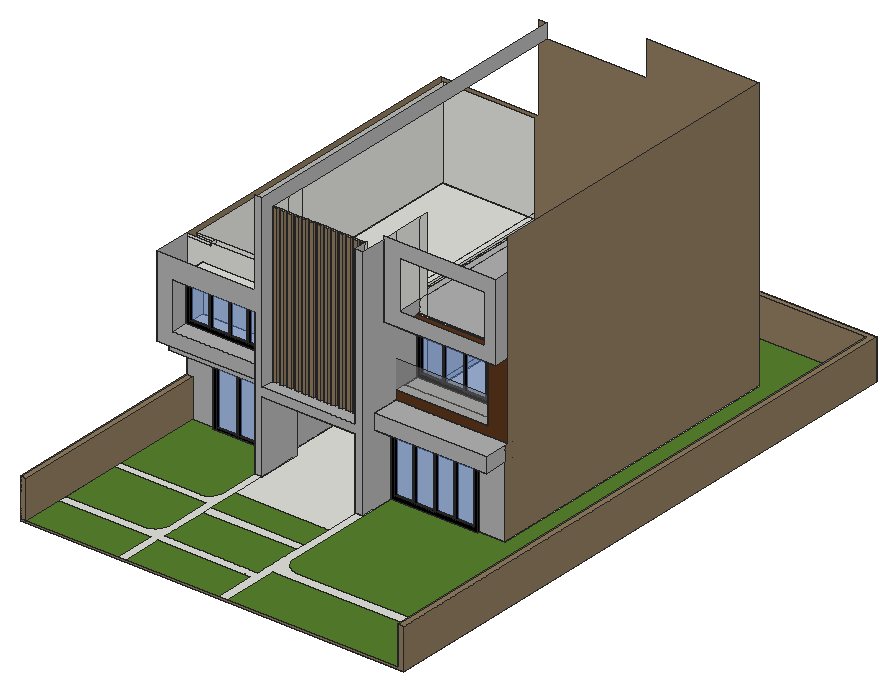
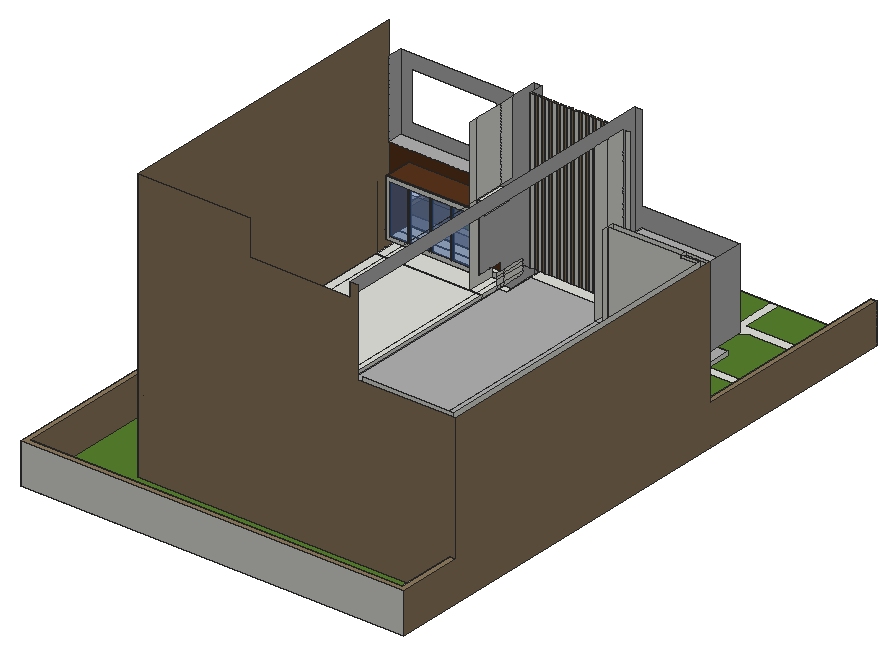
# SketchUp Ruby script. Lengths in inches.
U = 1.inch
M = Sketchup.active_model
def pt(a) = Geom::Point3d.new(a.map { |v| v * U })
def face(e, loops, mat)
  f = e.add_face(loops[0].map { |a| pt(a) })
  loops[1..].each { |l| e.add_face(l.map { |a| pt(a) }).erase! }
  f.material = f.back_material = mat if mat
  f
end
# faces: each face lists its corners as indices into pts; further lists are holes
def faces(e, pts, list, mat = nil) = list.each { |f| face(e, (f[0].is_a?(Array) ? f : [f]).map { |l| l.map { |i| pts[i] } }, mat) }
# xy, xz, yz: faces in a plane at the given z, y or x. An outline is a flat list of corners, or four numbers for a rectangle; further outlines are holes
def ring(l) = l.size == 4 ? [[l[0], l[1]], [l[2], l[1]], [l[2], l[3]], [l[0], l[3]]] : l.each_slice(2).to_a
def flat(e, list, mat, &to3) = list.each { |f| face(e, (f[0].is_a?(Array) ? f : [f]).map { |l| ring(l).map { |u, v| to3.(u, v) } }, mat) }
def xy(e, z, list, mat = nil) = flat(e, list, mat) { |x, y| [x, y, z] }
def xz(e, y, list, mat = nil) = flat(e, list, mat) { |x, z| [x, y, z] }
def yz(e, x, list, mat = nil) = flat(e, list, mat) { |y, z| [x, y, z] }
def lines(e, pts, list) = list.each { |a, b| e.add_line(pt(pts[a]), pt(pts[b])) }
# prism: a flat outline (further loops are holes) pulled along v
def prism(e, loops, v, mat = nil)
  f = face(e, loops, mat); d = Geom::Vector3d.new(v.map { |x| x * U })
  f.pushpull(f.normal.samedirection?(d) ? d.length : -d.length)
end
def box(e, o, s, mat = nil) = prism(e, [[o, [o[0] + s[0], o[1], o[2]], [o[0] + s[0], o[1] + s[1], o[2]], [o[0], o[1] + s[1], o[2]]]], [0, 0, s[2]], mat)
def at(x, y, z, deg = 0) = Geom::Transformation.translation(pt([x, y, z])) * Geom::Transformation.rotation(ORIGIN, Z_AXIS, deg.degrees)
def axes(o, x, y, z) = Geom::Transformation.new([*x, 0, *y, 0, *z, 0, *pt(o).to_a, 1])
def part(name) = M.definitions.add(name)
# library, detail: a bought-in or finely detailed component or shape, given as its bounding box
def library(name, o, s) = part(name).tap { |d| box(d.entities, o, s) }
def detail(e, o, s) = box(e.add_group.entities, o, s)
def put(e, d, t, mat = nil) = e.add_instance(d, t).tap { |i| i.material = mat if mat }
def group(e, t, mat = nil) = e.add_group.tap { |g| g.transformation = t; g.material = mat if mat }.entities
root = M.entities
M.materials.add("Niraj_Hair_Gray").color = [178, 178, 178]
M.materials.add("[0035_Tan]").color = [142, 122, 95]
M.materials.add("[0137_Black]").color = [0, 0, 0]
M.materials.add("[Grass Dark Green]").color = [87, 130, 45]
M.materials.add("[Translucent Glass Blue]").color = [100, 149, 237]
M.materials["[Translucent Glass Blue]"].alpha = 0.5
M.materials.add("[Translucent Glass Gray]").color = [128, 128, 128]
M.materials["[Translucent Glass Gray]"].alpha = 0.5
M.materials.add("[Wood Veneer 01]").color = [89, 52, 27]
xy(root,0,[[0,0,0,325.73,43.58,325.73,43.58,322.73,152.61,322.73,152.61,267.73,164.61,267.73,164.61,334.73,152.61,334.73,152.61,814.73,322.3125,814.73,322.3125,334.73,310.3125,334.73,310.3125,267.73,322.3125,267.73,322.3125,325.73,498,325.73,498,823.73,0,823.73,0,925.52,599.79,925.52,599.79,0],[152.61,267.73,164.61,289.73],[310.3125,267.73,322.3125,289.73],[152.61,289.73,164.61,325.73],[310.3125,289.73,322.3125,325.73],
  [43.58,322.73,152.61,325.73],[0,325.73,0,823.73,498,823.73,498,325.73,322.3125,325.73,322.3125,334.73,489,334.73,489,814.73,9,814.73,9,334.73,152.61,334.73,152.61,325.73],[152.61,325.73,164.61,334.73],[310.3125,325.73,322.3125,334.73],[9,334.73,152.61,814.73],
  [322.3125,334.73,489,814.73]])
xy(root,3,[[152.61,0,164.5625,0,164.5625,63.91,310.3125,63.91,310.3125,0,322.96,0,322.96,90.65,590.79,90.65,590.79,105.17,349.55,105.17,346.08,105.39,342.67,106.07,339.38,107.19,336.26,108.73,333.37,110.66,330.75,112.96,328.46,115.57,326.52,118.46,324.99,121.58,323.87,124.88,323.1875,128.29,322.96,131.76,322.96,267.73,310.3125,267.73,310.3125,76.4,164.5625,76.4,164.5625,267.73,152.61,267.73,152.61,206.62,152.43,203.89,151.9,201.2,151.02,198.61,149.8125,196.16,148.29,193.89,146.49,191.83,144.43,190.03,142.16,188.51,139.7,187.3,137.11,186.42,134.43,185.89,131.7,185.71,9,185.71,9,172.8,152.61,172.8,152.61,104.46,152.39,101.12,151.74,97.83,150.66,94.65,149.18,91.64,147.3125,88.85,145.1,86.33,142.58,84.11,139.79,82.25,136.78,80.77,133.6,79.6875,130.31,79.03,126.96,78.8125,9,78.8125,9,63.91,152.61,63.91],[306.22,63.75,310.3125,63.91,300.72,63.91,302.13,63.82],[164.5625,152.8,310.3125,166.42],[164.5625,215.1875,310.3125,215.1875,310.3125,334.73,322.3125,334.73,322.3125,814.73,152.61,814.73,152.61,334.73,164.61,334.73,164.61,267.73,164.5625,267.73],[322.3125,322.73,457.59,325.73]])
xy(root,3,[[9,0,152.61,63.91],[164.5625,0,310.3125,0,310.3125,63.91,306.22,63.75,302.13,63.82,300.72,63.91,164.5625,63.91],[322.96,0,590.79,90.65],[164.5625,76.4,310.3125,152.8],[9,78.8125,126.96,78.8125,130.31,79.03,133.6,79.6875,136.78,80.77,139.79,82.25,142.58,84.11,145.1,86.33,147.3125,88.85,149.18,91.64,150.66,94.65,151.74,97.83,152.39,101.12,152.61,104.46,152.61,172.8,9,172.8],
  [349.55,105.17,590.79,105.17,590.79,916.52,9,916.52,9,823.73,498,823.73,498,325.73,457.59,325.73,457.59,322.73,322.3125,322.73,322.3125,267.73,322.96,267.73,322.96,131.76,323.1875,128.29,323.87,124.88,324.99,121.58,326.52,118.46,328.46,115.57,330.75,112.96,333.37,110.66,336.26,108.73,339.38,107.19,342.67,106.07,346.08,105.39],[164.5625,166.42,310.3125,215.1875],[9,185.71,131.7,185.71,134.43,185.89,137.11,186.42,139.7,187.3,142.16,188.51,144.43,190.03,146.49,191.83,148.29,193.89,149.8125,196.16,151.02,198.61,151.9,201.2,152.43,203.89,152.61,206.62,152.61,322.73,43.58,322.73,43.58,325.73,9,325.73]],"[Grass Dark Green]")
xy(root,6,[[49.58,322.73,81.37,325.73],[84.37,322.73,116.66,325.73],[119.66,322.73,146.61,325.73]],"[0137_Black]")
xy(root,9,[[328.3125,322.73,356.625,325.73],[359.625,322.73,389.95,325.73],[392.95,322.73,421.03,325.73],[424.03,322.73,451.59,325.73]],"[0137_Black]")
xy(root,63,[[0,0,9,325.73],[590.79,0,599.79,0,599.79,925.52,0,925.52,0,823.73,9,823.73,9,916.52,590.79,916.52]],"[0035_Tan]")
xy(root,107.16,[[49.58,322.73,81.37,325.73],[84.37,322.73,116.66,325.73],[119.66,322.73,146.61,325.73]],"[0137_Black]")
xy(root,108.75,[[328.3125,322.73,356.625,325.73],[359.625,322.73,389.95,325.73],[392.95,322.73,421.03,325.73],[424.03,322.73,451.59,325.73]],"[0137_Black]")
xy(root,113.16,[[43.58,322.73,152.61,325.73]])
xy(root,113.16,[[0,289.73,0,325.73,43.58,325.73,43.58,322.73,152.61,322.73,152.61,289.73]],"Niraj_Hair_Gray")
xy(root,113.5,[[322.3125,334.73,489,369.1]])
xy(root,114.5625,[[164.61,267.73,310.3125,289.73],[152.61,325.73,164.61,334.73],[310.3125,325.73,322.3125,334.73]])
xy(root,114.5625,[[164.61,289.73,164.61,334.73,152.61,334.73,152.61,814.73,322.3125,814.73,322.3125,334.73,310.3125,334.73,310.3125,289.73]],"Niraj_Hair_Gray")
xy(root,114.75,[[322.3125,322.73,457.59,325.73]])
xy(root,114.75,[[322.3125,289.73,322.3125,322.73,457.59,322.73,457.59,325.73,498,325.73,498,289.73]],"Niraj_Hair_Gray")
xy(root,120,[[322.3125,325.73,489,369.1],[9,334.73,151.88,814.73],[322.3125,369.1,489,814.73]])
xy(root,120,[[0,289.73,152.61,325.73]],"Niraj_Hair_Gray")
xy(root,128.125,[[165.47,286.73,172.3125,289.73],[176.97,286.73,183.8125,289.73],[188.47,286.73,195.3125,289.73],[199.97,286.73,206.8125,289.73],[211.47,286.73,218.3125,289.73],
  [222.97,286.73,229.8125,289.73],[234.47,286.73,241.3125,289.73],[245.97,286.73,252.8125,289.73],[257.47,286.73,264.3125,289.73],[268.97,286.73,275.8125,289.73],
  [280.47,286.73,287.3125,289.73],[291.97,286.73,298.8125,289.73],[303.47,286.73,310.3125,289.73]])
xy(root,128.125,[[164.61,267.73,310.3125,267.73,310.3125,286.73,303.47,286.73,303.47,289.73,298.8125,289.73,298.8125,286.73,291.97,286.73,291.97,289.73,287.3125,289.73,287.3125,286.73,280.47,286.73,280.47,289.73,275.8125,289.73,275.8125,286.73,268.97,286.73,268.97,289.73,264.3125,289.73,264.3125,286.73,257.47,286.73,257.47,289.73,252.8125,289.73,252.8125,286.73,245.97,286.73,245.97,289.73,241.3125,289.73,241.3125,286.73,234.47,286.73,234.47,289.73,229.8125,289.73,229.8125,286.73,222.97,286.73,222.97,289.73,218.3125,289.73,218.3125,286.73,211.47,286.73,211.47,289.73,206.8125,289.73,206.8125,286.73,199.97,286.73,199.97,289.73,195.3125,289.73,195.3125,286.73,188.47,286.73,188.47,289.73,183.8125,289.73,183.8125,286.73,176.97,286.73,176.97,289.73,172.3125,289.73,172.3125,286.73,165.47,286.73,165.47,289.73,164.61,289.73]],"Niraj_Hair_Gray")
xy(root,135.375,[[0,267.73,152.61,325.73]],"Niraj_Hair_Gray")
xy(root,137.94,[[322.3125,332.48,466.55,339.92],[322.3125,349.98,466.55,392.92]])
xy(root,137.94,[[322.3125,289.73,498,332.48]],"Niraj_Hair_Gray")
xy(root,151.32,[[322.3125,332.48,466.55,349.98],[322.3125,349.98,466.55,373.98],[322.3125,373.98,466.55,376.98]])
xy(root,157.07,[[24.625,294.04,152.61,297.04],[24.625,297.04,152.61,325.73]])
xy(root,157.07,[[24.625,267.73,152.61,294.04]],"Niraj_Hair_Gray")
xy(root,157.32,[[328.3125,373.98,362.38,376.98],[365.38,373.98,394.43,376.98],[397.43,373.98,429.41,376.98],[432.41,373.98,460.55,376.98]],"[0137_Black]")
xy(root,163.07,[[30.625,294.04,60.5,297.04],[63.5,294.04,91.1875,297.04],[94.1875,294.04,119.75,297.04],[122.75,294.04,146.61,297.04]],"[0137_Black]")
xy(root,223.39,[[30.625,294.04,60.5,297.04],[63.5,294.04,91.1875,297.04],[94.1875,294.04,119.75,297.04],[122.75,294.04,146.61,297.04]],"[0137_Black]")
xy(root,229.39,[[24.625,294.04,152.61,297.04],[24.625,297.04,152.61,325.73]])
xy(root,229.39,[[24.625,267.73,152.61,294.04]],"Niraj_Hair_Gray")
xy(root,234,[[328.3125,373.98,362.38,376.98],[365.38,373.98,394.43,376.98],[397.43,373.98,429.41,376.98],[432.41,373.98,460.55,376.98]],"[0137_Black]")
xy(root,240,[[322.3125,373.98,466.55,376.98]])
xy(root,240,[[322.3125,332.48,466.55,373.98]],"[Wood Veneer 01]")
xy(root,240.1,[[309.68,332.48,322.3125,379.48]])
xy(root,257.94,[[309.68,332.48,322.3125,379.48]])
xy(root,257.94,[[322.3125,308.48,498,332.48]],"Niraj_Hair_Gray")
xz(root,0,[[0,0,599.79,0,599.79,63,590.79,63,590.79,3,0,3],[0,3,9,63]],"[0035_Tan]")
xz(root,267.73,[[152.61,0,164.61,3],[310.3125,0,322.3125,3]])
xz(root,267.73,[[152.61,3,164.61,3,164.61,114.5625,310.3125,114.5625,310.3125,3,322.3125,3,322.3125,372.875,310.3125,372.875,310.3125,128.125,164.61,128.125,164.61,394.4375,152.61,394.4375,152.61,261.125,0,261.125,0,135.375,152.61,135.375,152.61,157.07,24.625,157.07,24.625,229.39,152.61,229.39]],"Niraj_Hair_Gray")
xz(root,286.73,[[165.47,128.125,172.3125,372.875],[176.97,128.125,183.8125,372.875],[188.47,128.125,195.3125,372.875],[199.97,128.125,206.8125,372.875],[211.47,128.125,218.3125,372.875],
  [222.97,128.125,229.8125,372.875],[234.47,128.125,241.3125,372.875],[245.97,128.125,252.8125,372.875],[257.47,128.125,264.3125,372.875],[268.97,128.125,275.8125,372.875],
  [280.47,128.125,287.3125,372.875],[291.97,128.125,298.8125,372.875],[303.47,128.125,310.3125,372.875]],"[0035_Tan]")
xz(root,289.73,[[153.97,128.125,160.8125,372.875],[165.47,128.125,172.3125,372.875],[176.97,128.125,183.8125,372.875],[188.47,128.125,195.3125,372.875],[199.97,128.125,206.8125,372.875],
  [211.47,128.125,218.3125,372.875],[222.97,128.125,229.8125,372.875],[234.47,128.125,241.3125,372.875],[245.97,128.125,252.8125,372.875],[257.47,128.125,264.3125,372.875],
  [268.97,128.125,275.8125,372.875],[280.47,128.125,287.3125,372.875],[291.97,128.125,298.8125,372.875],[303.47,128.125,310.3125,372.875]])
xz(root,289.73,[[0,113.16,152.61,120],[322.3125,114.75,498,137.94]],"Niraj_Hair_Gray")
xz(root,289.73,[[164.61,128.125,165.47,372.875],[172.3125,128.125,176.97,372.875],[183.8125,128.125,188.47,372.875],[195.3125,128.125,199.97,372.875],[206.8125,128.125,211.47,372.875],
  [218.3125,128.125,222.97,372.875],[229.8125,128.125,234.47,372.875],[241.3125,128.125,245.97,372.875],[252.8125,128.125,257.47,372.875],[264.3125,128.125,268.97,372.875],
  [275.8125,128.125,280.47,372.875],[287.3125,128.125,291.97,372.875],[298.8125,128.125,303.47,372.875]],"[0035_Tan]")
xz(root,294.04,[[[24.625,157.07,152.61,229.39],[30.625,163.07,60.5,223.39],[63.5,163.07,91.1875,223.39],[94.1875,163.07,119.75,223.39],[122.75,163.07,146.61,223.39]]],"[0137_Black]")
xz(root,297.04,[[[24.625,157.07,152.61,229.39],[30.625,163.07,60.5,223.39],[63.5,163.07,91.1875,223.39],[94.1875,163.07,119.75,223.39],[122.75,163.07,146.61,223.39]]])
xz(root,297.04,[[30.625,163.07,60.5,223.39],[63.5,163.07,91.1875,223.39],[94.1875,163.07,119.75,223.39],[122.75,163.07,146.61,223.39]],"[Translucent Glass Blue]")
xz(root,308.48,[[[322.3125,257.94,498,377.94],[346.71,279.54,480.7,355.07]]],"Niraj_Hair_Gray")
xz(root,322.73,[[43.58,0,152.61,3]])
xz(root,322.73,[[[43.58,3,152.61,113.16],[84.37,6,116.66,107.16],[49.58,6,81.37,107.16],[119.66,6,146.61,107.16]],[[322.3125,3,457.59,114.75],[359.625,9,389.95,108.75],[328.3125,9,356.625,108.75],[392.95,9,421.03,108.75],[424.03,9,451.59,108.75]]],"[0137_Black]")
xz(root,325.73,[[[43.58,0,152.61,113.16],[84.37,6,116.66,107.16],[49.58,6,81.37,107.16],[119.66,6,146.61,107.16]],[322.3125,0,498,3],[[322.3125,3,457.59,114.75],[359.625,9,389.95,108.75],[328.3125,9,356.625,108.75],[392.95,9,421.03,108.75],[424.03,9,451.59,108.75]],[0,113.16,152.61,120],[322.3125,114.75,489,120],
  [489,114.75,498,120],[322.3125,120,498,132.82],[0,135.375,0,257.3125,38.3125,257.3125,38.3125,261.125,152.61,261.125,152.61,229.39,24.625,229.39,24.625,157.07,152.61,157.07,152.61,135.375],[0,257.3125,38.3125,261.125]])
xz(root,325.73,[[9,3,43.58,3,43.58,113.16,0,113.16,0,63,9,63],[457.59,3,498,114.75],[0,120,152.61,135.375]],"Niraj_Hair_Gray")
xz(root,325.73,[[49.58,6,81.37,107.16],[84.37,6,116.66,107.16],[119.66,6,146.61,107.16],[328.3125,9,356.625,108.75],[359.625,9,389.95,108.75],
  [392.95,9,421.03,108.75],[424.03,9,451.59,108.75]],"[Translucent Glass Blue]")
xz(root,332.48,[[322.3125,151.32,466.55,195.66]],"[Translucent Glass Gray]")
xz(root,332.48,[[322.3125,137.94,498,137.94,498,257.94,309.68,257.94,309.68,240.1,322.3125,240.1,322.3125,240,466.55,240,466.55,151.32,322.3125,151.32]],"[Wood Veneer 01]")
xz(root,334.73,[[9,0,9,120,151.88,120,151.88,261.125,152.61,261.125,152.61,0],[152.61,0,164.61,3],[310.3125,0,322.3125,3],[322.3125,0,489,113.5],[152.61,3,164.61,114.5625],
  [9,120,9,257.3125,38.3125,257.3125,38.3125,261.125,151.88,261.125,151.88,120],[9,257.3125,38.3125,261.125]])
xz(root,334.73,[[310.3125,3,322.3125,114.5625]],"Niraj_Hair_Gray")
xz(root,349.98,[[322.3125,137.94,466.55,151.32]])
xz(root,369.1,[[322.3125,113.5,489,120]])
xz(root,373.98,[[[322.3125,151.32,466.55,240],[328.3125,157.32,362.38,234],[397.43,157.32,429.41,234],[365.38,157.32,394.43,234],[432.41,157.32,460.55,234]]],"[0137_Black]")
xz(root,376.98,[[[322.3125,151.32,466.55,240],[328.3125,157.32,362.38,234],[397.43,157.32,429.41,234],[365.38,157.32,394.43,234],[432.41,157.32,460.55,234]]])
xz(root,376.98,[[328.3125,157.32,362.38,234],[365.38,157.32,394.43,234],[397.43,157.32,429.41,234],[432.41,157.32,460.55,234]],"[Translucent Glass Blue]")
xz(root,379.48,[[309.68,240.1,322.3125,257.94]])
xz(root,814.73,[[9,0,152.61,120],[152.61,0,322.3125,3],[322.3125,0,489,120],[152.61,114.5625,322.3125,120],[9,120,151.88,261.125]])
xz(root,814.73,[[152.61,3,322.3125,114.5625]],"Niraj_Hair_Gray")
xz(root,823.73,[[9,3,9,63,0,63,0,261.125,152.61,261.125,152.61,394.4375,164.61,394.4375,164.61,372.875,322.3125,372.875,322.3125,428.22,498,428.22,498,3]],"[0035_Tan]")
xz(root,916.52,[[9,3,590.79,63]],"[0035_Tan]")
xz(root,925.52,[[0,0,599.79,63]])
yz(root,0,[[289.73,113.16,325.73,120]])
yz(root,0,[[267.73,135.375,325.73,261.125]],"Niraj_Hair_Gray")
yz(root,0,[[0,0,0,63,325.73,63,325.73,261.125,823.73,261.125,823.73,63,925.52,63,925.52,0]],"[0035_Tan]")
yz(root,9,[[334.73,0,814.73,120],[823.73,3,916.52,63],[334.73,120,814.73,261.125]])
yz(root,9,[[0,3,325.73,63]],"[0035_Tan]")
yz(root,24.625,[[294.04,157.07,297.04,229.39],[297.04,157.07,325.73,229.39]])
yz(root,24.625,[[267.73,157.07,294.04,229.39]],"Niraj_Hair_Gray")
yz(root,30.625,[[294.04,163.07,297.04,223.39]],"[0137_Black]")
yz(root,38.3125,[[325.73,257.3125,334.73,261.125]])
yz(root,43.58,[[322.73,0,325.73,3]])
yz(root,43.58,[[322.73,3,325.73,113.16]],"[0137_Black]")
yz(root,49.58,[[322.73,6,325.73,107.16]],"[0137_Black]")
yz(root,60.5,[[294.04,163.07,297.04,223.39]],"[0137_Black]")
yz(root,63.5,[[294.04,163.07,297.04,223.39]],"[0137_Black]")
yz(root,81.37,[[322.73,6,325.73,107.16]],"[0137_Black]")
yz(root,84.37,[[322.73,6,325.73,107.16]],"[0137_Black]")
yz(root,91.1875,[[294.04,163.07,297.04,223.39]],"[0137_Black]")
yz(root,94.1875,[[294.04,163.07,297.04,223.39]],"[0137_Black]")
yz(root,116.66,[[322.73,6,325.73,107.16]],"[0137_Black]")
yz(root,119.66,[[322.73,6,325.73,107.16]],"[0137_Black]")
yz(root,119.75,[[294.04,163.07,297.04,223.39]],"[0137_Black]")
yz(root,122.75,[[294.04,163.07,297.04,223.39]],"[0137_Black]")
yz(root,146.61,[[322.73,6,325.73,107.16],[294.04,163.07,297.04,223.39]],"[0137_Black]")
yz(root,152.61,[[267.73,0,289.73,3],[289.73,0,322.73,3],[322.73,0,325.73,113.16],[325.73,0,334.73,114.5625],[334.73,0,814.73,3],
  [289.73,113.16,325.73,114.5625],[289.73,114.5625,325.73,120],[325.73,114.5625,334.73,120],[334.73,114.5625,814.73,120],[325.73,120,334.73,128.125],
  [325.73,128.125,334.73,128.125,334.73,261.125,325.73,261.125,325.73,229.39,297.04,229.39,297.04,157.07,325.73,157.07],[334.73,128.125,344.66,261.125],[267.73,135.375,325.73,157.07],[267.73,157.07,294.04,229.39],[294.04,157.07,297.04,229.39]])
yz(root,152.61,[[267.73,3,267.73,135.375,325.73,135.375,325.73,120,289.73,120,289.73,113.16,322.73,113.16,322.73,3],[334.73,3,814.73,114.5625]],"Niraj_Hair_Gray")
yz(root,164.61,[[267.73,0,289.73,3],[289.73,0,325.73,3],[325.73,0,334.73,3],[289.73,128.125,319.91,372.875],[319.91,128.125,344.66,372.875]])
yz(root,164.61,[[267.73,3,334.73,114.5625],[267.73,128.125,289.73,128.125,289.73,372.875,823.73,372.875,823.73,394.4375,267.73,394.4375]],"Niraj_Hair_Gray")
yz(root,165.47,[[286.73,128.125,289.73,372.875]])
yz(root,172.3125,[[286.73,128.125,289.73,372.875]],"[0035_Tan]")
yz(root,176.97,[[286.73,128.125,289.73,372.875]],"[0035_Tan]")
yz(root,183.8125,[[286.73,128.125,289.73,372.875]],"[0035_Tan]")
yz(root,188.47,[[286.73,128.125,289.73,372.875]],"[0035_Tan]")
yz(root,195.3125,[[286.73,128.125,289.73,372.875]],"[0035_Tan]")
yz(root,199.97,[[286.73,128.125,289.73,372.875]],"[0035_Tan]")
yz(root,206.8125,[[286.73,128.125,289.73,372.875]],"[0035_Tan]")
yz(root,211.47,[[286.73,128.125,289.73,372.875]],"[0035_Tan]")
yz(root,218.3125,[[286.73,128.125,289.73,372.875]],"[0035_Tan]")
yz(root,222.97,[[286.73,128.125,289.73,372.875]],"[0035_Tan]")
yz(root,229.8125,[[286.73,128.125,289.73,372.875]],"[0035_Tan]")
yz(root,234.47,[[286.73,128.125,289.73,372.875]],"[0035_Tan]")
yz(root,241.3125,[[286.73,128.125,289.73,372.875]],"[0035_Tan]")
yz(root,245.97,[[286.73,128.125,289.73,372.875]],"[0035_Tan]")
yz(root,252.8125,[[286.73,128.125,289.73,372.875]],"[0035_Tan]")
yz(root,257.47,[[286.73,128.125,289.73,372.875]],"[0035_Tan]")
yz(root,264.3125,[[286.73,128.125,289.73,372.875]],"[0035_Tan]")
yz(root,268.97,[[286.73,128.125,289.73,372.875]],"[0035_Tan]")
yz(root,275.8125,[[286.73,128.125,289.73,372.875]],"[0035_Tan]")
yz(root,280.47,[[286.73,128.125,289.73,372.875]],"[0035_Tan]")
yz(root,287.3125,[[286.73,128.125,289.73,372.875]],"[0035_Tan]")
yz(root,291.97,[[286.73,128.125,289.73,372.875]],"[0035_Tan]")
yz(root,298.8125,[[286.73,128.125,289.73,372.875]],"[0035_Tan]")
yz(root,303.47,[[286.73,128.125,289.73,372.875]],"[0035_Tan]")
yz(root,309.68,[[332.48,240.1,379.48,257.94]])
yz(root,310.3125,[[267.73,0,289.73,3],[289.73,0,325.73,3],[325.73,0,334.73,3],[286.73,128.125,289.73,372.875]])
yz(root,310.3125,[[267.73,3,334.73,114.5625],[267.73,128.125,286.73,372.875]],"Niraj_Hair_Gray")
yz(root,322.3125,[[267.73,0,289.73,3],[289.73,0,325.73,3],[325.73,0,334.73,114.5625],[334.73,0,814.73,3],[322.73,3,325.73,114.5625],
  [334.73,113.5,369.1,114.5625],[322.73,114.5625,325.73,114.75],[325.73,114.5625,334.73,114.75],[334.73,114.5625,334.73,114.75,339.92,114.75,339.92,120,369.1,120,369.1,114.5625],[369.1,114.5625,814.73,120],
  [289.73,114.75,325.73,120],[325.73,114.75,334.73,120],[334.73,114.75,339.92,120],[289.73,120,325.73,128.125],[325.73,120,339.92,128.125],
  [289.73,128.125,325.73,132.82],[325.73,128.125,339.92,132.82],[289.73,132.82,325.73,137.94],[325.73,132.82,339.92,137.94],[349.98,137.94,349.98,151.32,376.98,151.32,376.98,240,379.48,240,379.48,257.94,392.92,257.94,392.92,137.94],
  [373.98,151.32,376.98,240],[308.48,257.94,332.48,372.875],[332.48,257.94,379.48,372.875],[379.48,257.94,392.92,372.875]])
yz(root,322.3125,[[267.73,3,322.73,3,322.73,114.75,289.73,114.75,289.73,137.94,332.48,137.94,332.48,151.32,373.98,151.32,373.98,240,332.48,240,332.48,240.1,379.48,240.1,379.48,257.94,308.48,257.94,308.48,372.875,267.73,372.875],[334.73,3,334.73,113.5,369.1,113.5,369.1,114.5625,814.73,114.5625,814.73,3]],"Niraj_Hair_Gray")
yz(root,328.3125,[[322.73,9,325.73,108.75],[373.98,157.32,376.98,234]],"[0137_Black]")
yz(root,356.625,[[322.73,9,325.73,108.75]],"[0137_Black]")
yz(root,359.625,[[322.73,9,325.73,108.75]],"[0137_Black]")
yz(root,362.38,[[373.98,157.32,376.98,234]],"[0137_Black]")
yz(root,365.38,[[373.98,157.32,376.98,234]],"[0137_Black]")
yz(root,389.95,[[322.73,9,325.73,108.75]],"[0137_Black]")
yz(root,392.95,[[322.73,9,325.73,108.75]],"[0137_Black]")
yz(root,394.43,[[373.98,157.32,376.98,234]],"[0137_Black]")
yz(root,397.43,[[373.98,157.32,376.98,234]],"[0137_Black]")
yz(root,421.03,[[322.73,9,325.73,108.75]],"[0137_Black]")
yz(root,424.03,[[322.73,9,325.73,108.75]],"[0137_Black]")
yz(root,429.41,[[373.98,157.32,376.98,234]],"[0137_Black]")
yz(root,432.41,[[373.98,157.32,376.98,234]],"[0137_Black]")
yz(root,451.59,[[322.73,9,325.73,108.75]],"[0137_Black]")
yz(root,457.59,[[322.73,3,325.73,114.75]],"[0137_Black]")
yz(root,460.55,[[373.98,157.32,376.98,234]],"[0137_Black]")
yz(root,466.55,[[373.98,151.32,376.98,240]])
yz(root,466.55,[[332.48,151.32,373.98,240]],"[Wood Veneer 01]")
yz(root,489,[[334.73,0,334.73,113.5,369.1,113.5,369.1,120,814.73,120,814.73,0]])
yz(root,498,[[325.73,0,823.73,3]])
yz(root,498,[[289.73,114.75,325.73,137.94],[308.48,257.94,332.48,377.94]],"Niraj_Hair_Gray")
yz(root,498,[[325.73,3,823.73,3,823.73,428.22,332.48,428.22,332.48,137.94,325.73,137.94]],"[0035_Tan]")
yz(root,590.79,[[0,3,916.52,63]],"[0035_Tan]")
yz(root,599.79,[[0,0,925.52,63]],"[0035_Tan]")
p = [[164.61,289.73,128.125],[160.8125,289.73,128.125],[152.61,344.66,128.125],[152.61,814.73,128.125],[164.61,344.66,128.125],[164.61,814.73,128.125],
  [489,334.73,113.5],[489,334.73,120],[310.3125,289.73,128.125],[322.3125,289.73,128.125],[322.3125,339.92,114.75],[498,339.92,114.75],
  [498,339.92,137.94],[466.55,339.92,137.94],[322.3125,339.92,128.125],[322.3125,814.73,128.125],[466.55,392.92,137.94],[466.55,392.92,240],
  [322.3125,814.73,257.94],[322.3125,392.92,257.94],[489,814.73,120],[489,823.73,120],[0,325.73,3],[9,325.73,3]]
lines(root,p,[[0,1],[2,3],[2,4],[4,5],[6,7],[8,9],[10,11],[12,13],[14,15],[16,17],[18,19],[20,21],
  [22,23]])
